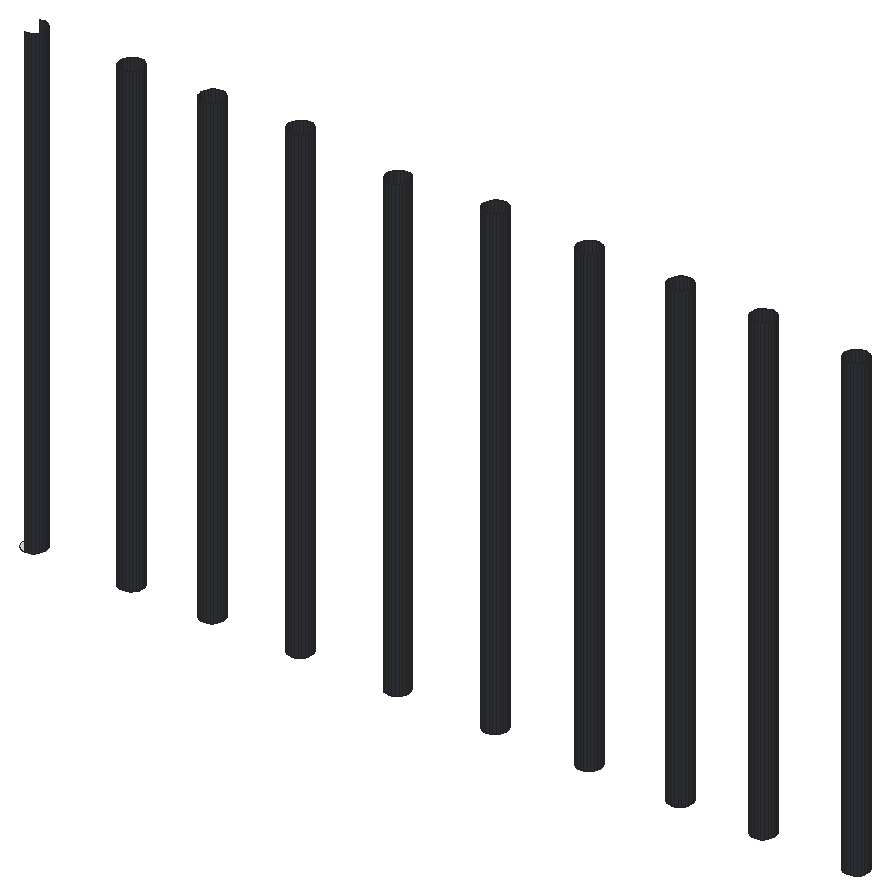
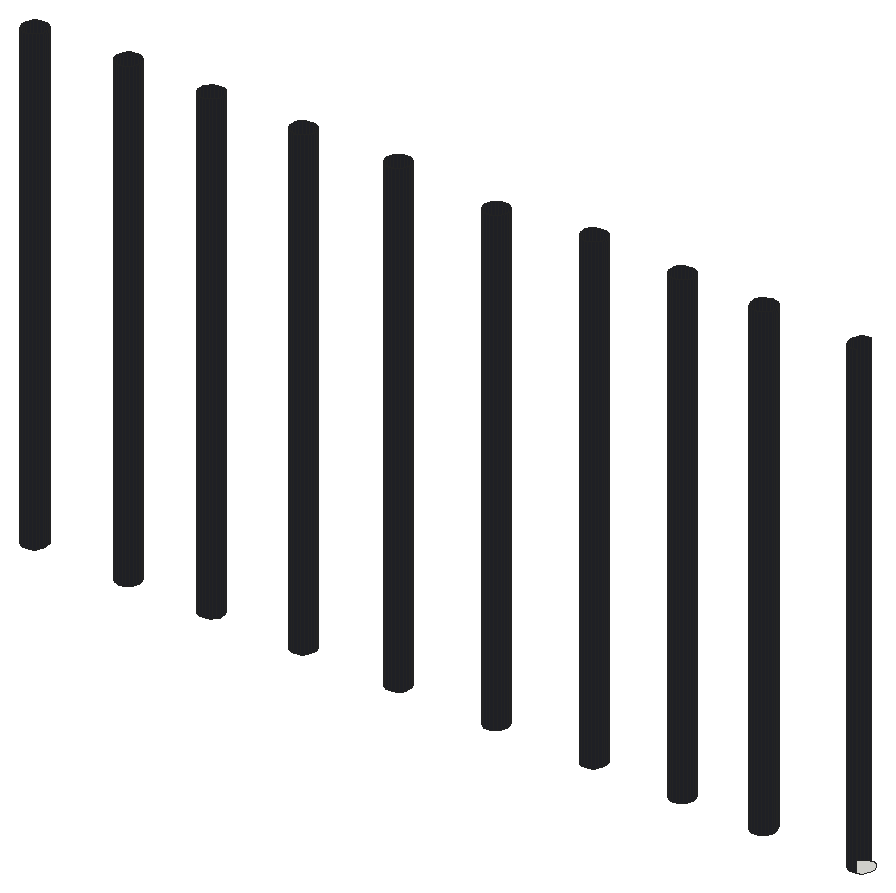
# SketchUp Ruby script. Lengths in inches.
U = 1.inch
M = Sketchup.active_model
def pt(a) = Geom::Point3d.new(a.map { |v| v * U })
def face(e, loops, mat)
  f = e.add_face(loops[0].map { |a| pt(a) })
  loops[1..].each { |l| e.add_face(l.map { |a| pt(a) }).erase! }
  f.material = f.back_material = mat if mat
  f
end
# faces: each face lists its corners as indices into pts; further lists are holes
def faces(e, pts, list, mat = nil) = list.each { |f| face(e, (f[0].is_a?(Array) ? f : [f]).map { |l| l.map { |i| pts[i] } }, mat) }
# xy, xz, yz: faces in a plane at the given z, y or x. An outline is a flat list of corners, or four numbers for a rectangle; further outlines are holes
def ring(l) = l.size == 4 ? [[l[0], l[1]], [l[2], l[1]], [l[2], l[3]], [l[0], l[3]]] : l.each_slice(2).to_a
def flat(e, list, mat, &to3) = list.each { |f| face(e, (f[0].is_a?(Array) ? f : [f]).map { |l| ring(l).map { |u, v| to3.(u, v) } }, mat) }
def xy(e, z, list, mat = nil) = flat(e, list, mat) { |x, y| [x, y, z] }
def xz(e, y, list, mat = nil) = flat(e, list, mat) { |x, z| [x, y, z] }
def yz(e, x, list, mat = nil) = flat(e, list, mat) { |y, z| [x, y, z] }
def lines(e, pts, list) = list.each { |a, b| e.add_line(pt(pts[a]), pt(pts[b])) }
# prism: a flat outline (further loops are holes) pulled along v
def prism(e, loops, v, mat = nil)
  f = face(e, loops, mat); d = Geom::Vector3d.new(v.map { |x| x * U })
  f.pushpull(f.normal.samedirection?(d) ? d.length : -d.length)
end
def box(e, o, s, mat = nil) = prism(e, [[o, [o[0] + s[0], o[1], o[2]], [o[0] + s[0], o[1] + s[1], o[2]], [o[0], o[1] + s[1], o[2]]]], [0, 0, s[2]], mat)
def at(x, y, z, deg = 0) = Geom::Transformation.translation(pt([x, y, z])) * Geom::Transformation.rotation(ORIGIN, Z_AXIS, deg.degrees)
def axes(o, x, y, z) = Geom::Transformation.new([*x, 0, *y, 0, *z, 0, *pt(o).to_a, 1])
def part(name) = M.definitions.add(name)
# library, detail: a bought-in or finely detailed component or shape, given as its bounding box
def library(name, o, s) = part(name).tap { |d| box(d.entities, o, s) }
def detail(e, o, s) = box(e.add_group.entities, o, s)
def put(e, d, t, mat = nil) = e.add_instance(d, t).tap { |i| i.material = mat if mat }
def group(e, t, mat = nil) = e.add_group.tap { |g| g.transformation = t; g.material = mat if mat }.entities
root = M.entities
M.materials.add("[Formica Laminate Dark]").color = [50, 53, 60]
xy(root,1179.9375,[[1326.55,797.03,1324.75,797.27,1323.08,797.96,1321.64,799.06,1320.54,800.5,1319.84,802.17,1319.61,803.97,1319.84,805.77,1320.54,807.4375,1321.64,808.875,1323.08,809.98,1324.75,810.67,1326.55,810.91,1328.34,810.67,1330.01,809.98,1331.45,808.875,1332.55,807.4375,1333.25,805.77,1333.48,803.97,1333.25,802.17,1332.55,800.5,1331.45,799.06,1330.01,797.96,1328.34,797.27],[1386.05,797.03,1384.25,797.27,1382.58,797.96,1381.14,799.06,1380.04,800.5,1379.34,802.17,1379.11,803.97,1379.34,805.77,1380.04,807.4375,1381.14,808.875,1382.58,809.98,1384.25,810.67,1386.05,810.91,1387.84,810.67,1389.51,809.98,1390.95,808.875,1392.05,807.4375,1392.75,805.77,1392.98,803.97,1392.75,802.17,1392.05,800.5,1390.95,799.06,1389.51,797.96,1387.84,797.27],[1435.55,797.03,1433.75,797.27,1432.08,797.96,1430.64,799.06,1429.54,800.5,1428.84,802.17,1428.61,803.97,1428.84,805.77,1429.54,807.4375,1430.64,808.875,1432.08,809.98,1433.75,810.67,1435.55,810.91,1437.34,810.67,1439.01,809.98,1440.45,808.875,1441.55,807.4375,1442.25,805.77,1442.48,803.97,1442.25,802.17,1441.55,800.5,1440.45,799.06,1439.01,797.96,1437.34,797.27],[1489.3,797.03,1487.5,797.27,1485.83,797.96,1484.39,799.06,1483.29,800.5,1482.59,802.17,1482.36,803.97,1482.59,805.77,1483.29,807.4375,1484.39,808.875,1485.83,809.98,1487.5,810.67,1489.3,810.91,1491.09,810.67,1492.76,809.98,1494.2,808.875,1495.3,807.4375,1496,805.77,1496.23,803.97,1496,802.17,1495.3,800.5,1494.2,799.06,1492.76,797.96,1491.09,797.27],[1548.73,797.03,1546.9375,797.27,1545.26,797.96,1543.83,799.06,1542.73,800.5,1542.03,802.17,1541.8,803.97,1542.03,805.77,1542.73,807.4375,1543.83,808.875,1545.26,809.98,1546.9375,810.67,1548.73,810.91,1550.53,810.67,1552.2,809.98,1553.64,808.875,1554.74,807.4375,1555.43,805.77,1555.67,803.97,1555.43,802.17,1554.74,800.5,1553.64,799.06,1552.2,797.96,1550.53,797.27],
  [1608.3,797.03,1606.5,797.27,1604.83,797.96,1603.39,799.06,1602.29,800.5,1601.59,802.17,1601.36,803.97,1601.59,805.77,1602.29,807.4375,1603.39,808.875,1604.83,809.98,1606.5,810.67,1608.3,810.91,1610.09,810.67,1611.76,809.98,1613.2,808.875,1614.3,807.4375,1615,805.77,1615.23,803.97,1615,802.17,1614.3,800.5,1613.2,799.06,1611.76,797.96,1610.09,797.27],[1665.86,797.03,1664.0625,797.27,1662.39,797.96,1660.95,799.06,1659.85,800.5,1659.16,802.17,1658.92,803.97,1659.16,805.77,1659.85,807.4375,1660.95,808.875,1662.39,809.98,1664.0625,810.67,1665.86,810.91,1667.65,810.67,1669.33,809.98,1670.76,808.875,1671.87,807.4375,1672.56,805.77,1672.8,803.97,1672.56,802.17,1671.87,800.5,1670.76,799.06,1669.33,797.96,1667.65,797.27],[1721.48,797.03,1719.6875,797.27,1718.01,797.96,1716.58,799.06,1715.48,800.5,1714.78,802.17,1714.55,803.97,1714.78,805.77,1715.48,807.4375,1716.58,808.875,1718.01,809.98,1719.6875,810.67,1721.48,810.91,1723.28,810.67,1724.95,809.98,1726.39,808.875,1727.49,807.4375,1728.18,805.77,1728.42,803.97,1728.18,802.17,1727.49,800.5,1726.39,799.06,1724.95,797.96,1723.28,797.27],[1772.17,797.03,1770.375,797.27,1768.7,797.96,1767.27,799.06,1766.16,800.5,1765.47,802.17,1765.23,803.97,1765.47,805.77,1766.16,807.4375,1767.27,808.875,1768.7,809.98,1770.375,810.67,1772.17,810.91,1773.97,810.67,1775.64,809.98,1777.08,808.875,1778.18,807.4375,1778.87,805.77,1779.11,803.97,1778.87,802.17,1778.18,800.5,1777.08,799.06,1775.64,797.96,1773.97,797.27],[1828.92,797.03,1827.125,797.27,1825.45,797.96,1824.02,799.06,1822.91,800.5,1822.22,802.17,1821.98,803.97,1822.22,805.77,1822.91,807.4375,1824.02,808.875,1825.45,809.98,1827.125,810.67,1828.92,810.91,1830.72,810.67,1832.39,809.98,1833.83,808.875,1834.93,807.4375,1835.62,805.77,1835.86,803.97,1835.62,802.17,1834.93,800.5,1833.83,799.06,1832.39,797.96,1830.72,797.27]])
p = [[1326.55,797.03,1179.9375],[1328.34,797.27,1179.9375],[1328.34,797.27,1464.6875],[1326.55,797.03,1464.6875],[1384.25,797.27,1179.9375],[1386.05,797.03,1179.9375],
  [1386.05,797.03,1464.6875],[1384.25,797.27,1464.6875],[1387.84,797.27,1179.9375],[1387.84,797.27,1464.6875],[1433.75,797.27,1179.9375],[1435.55,797.03,1179.9375],
  [1435.55,797.03,1464.6875],[1433.75,797.27,1464.6875],[1437.34,797.27,1179.9375],[1437.34,797.27,1464.6875],[1487.5,797.27,1179.9375],[1489.3,797.03,1179.9375],
  [1489.3,797.03,1466.5],[1487.5,797.27,1466.5],[1491.09,797.27,1179.9375],[1491.09,797.27,1466.5],[1546.9375,797.27,1179.9375],[1548.73,797.03,1179.9375],
  [1548.73,797.03,1460],[1546.9375,797.27,1460],[1550.53,797.27,1179.9375],[1550.53,797.27,1460],[1606.5,797.27,1179.9375],[1608.3,797.03,1179.9375],
  [1608.3,797.03,1464.6875],[1606.5,797.27,1464.6875],[1610.09,797.27,1179.9375],[1610.09,797.27,1464.6875],[1664.0625,797.27,1179.9375],[1665.86,797.03,1179.9375],
  [1665.86,797.03,1462.7],[1664.0625,797.27,1462.7],[1667.65,797.27,1179.9375],[1667.65,797.27,1462.7],[1719.6875,797.27,1179.9375],[1721.48,797.03,1179.9375],
  [1721.48,797.03,1462.7],[1719.6875,797.27,1462.7],[1723.28,797.27,1179.9375],[1723.28,797.27,1462.7],[1770.375,797.27,1179.9375],[1772.17,797.03,1179.9375],
  [1772.17,797.03,1462.7],[1770.375,797.27,1462.7],[1773.97,797.27,1179.9375],[1773.97,797.27,1462.7],[1827.125,797.27,1179.9375],[1828.92,797.03,1179.9375],
  [1828.92,797.03,1460.3125],[1827.125,797.27,1460.3125],[1830.72,797.27,1179.9375],[1830.72,797.27,1460.3125],[1330.01,797.96,1179.9375],[1330.01,797.96,1464.6875],
  [1382.58,797.96,1179.9375],[1382.58,797.96,1464.6875],[1389.51,797.96,1179.9375],[1389.51,797.96,1464.6875],[1432.08,797.96,1179.9375],[1432.08,797.96,1464.6875],
  [1439.01,797.96,1179.9375],[1439.01,797.96,1464.6875],[1485.83,797.96,1179.9375],[1485.83,797.96,1466.5],[1492.76,797.96,1179.9375],[1492.76,797.96,1466.5],
  [1545.26,797.96,1179.9375],[1545.26,797.96,1460],[1552.2,797.96,1179.9375],[1552.2,797.96,1460],[1604.83,797.96,1179.9375],[1604.83,797.96,1464.6875],
  [1611.76,797.96,1179.9375],[1611.76,797.96,1464.6875],[1662.39,797.96,1179.9375],[1662.39,797.96,1462.7],[1669.33,797.96,1179.9375],[1669.33,797.96,1462.7],
  [1718.01,797.96,1179.9375],[1718.01,797.96,1462.7],[1724.95,797.96,1179.9375],[1724.95,797.96,1462.7],[1768.7,797.96,1179.9375],[1768.7,797.96,1462.7],
  [1775.64,797.96,1179.9375],[1775.64,797.96,1462.7],[1825.45,797.96,1179.9375],[1825.45,797.96,1460.3125],[1832.39,797.96,1179.9375],[1832.39,797.96,1460.3125],
  [1331.45,799.06,1179.9375],[1331.45,799.06,1464.6875],[1381.14,799.06,1179.9375],[1381.14,799.06,1464.6875],[1390.95,799.06,1179.9375],[1390.95,799.06,1464.6875],
  [1430.64,799.06,1179.9375],[1430.64,799.06,1464.6875],[1440.45,799.06,1179.9375],[1440.45,799.06,1464.6875],[1484.39,799.06,1179.9375],[1484.39,799.06,1466.5],
  [1494.2,799.06,1179.9375],[1494.2,799.06,1466.5],[1543.83,799.06,1179.9375],[1543.83,799.06,1460],[1553.64,799.06,1179.9375],[1553.64,799.06,1460],
  [1603.39,799.06,1179.9375],[1603.39,799.06,1464.6875],[1613.2,799.06,1179.9375],[1613.2,799.06,1464.6875],[1660.95,799.06,1179.9375],[1660.95,799.06,1462.7],
  [1670.76,799.06,1179.9375],[1670.76,799.06,1462.7],[1716.58,799.06,1179.9375],[1716.58,799.06,1462.7],[1726.39,799.06,1179.9375],[1726.39,799.06,1462.7],
  [1767.27,799.06,1179.9375],[1767.27,799.06,1462.7],[1777.08,799.06,1179.9375],[1777.08,799.06,1462.7],[1824.02,799.06,1179.9375],[1824.02,799.06,1460.3125],
  [1833.83,799.06,1179.9375],[1833.83,799.06,1460.3125],[1332.55,800.5,1179.9375],[1332.55,800.5,1464.6875],[1380.04,800.5,1179.9375],[1380.04,800.5,1464.6875],
  [1392.05,800.5,1179.9375],[1392.05,800.5,1464.6875],[1429.54,800.5,1179.9375],[1429.54,800.5,1464.6875],[1441.55,800.5,1179.9375],[1441.55,800.5,1464.6875],
  [1483.29,800.5,1179.9375],[1483.29,800.5,1466.5],[1495.3,800.5,1179.9375],[1495.3,800.5,1466.5],[1542.73,800.5,1179.9375],[1542.73,800.5,1460],
  [1554.74,800.5,1179.9375],[1554.74,800.5,1460],[1602.29,800.5,1179.9375],[1602.29,800.5,1464.6875],[1614.3,800.5,1179.9375],[1614.3,800.5,1464.6875],
  [1659.85,800.5,1179.9375],[1659.85,800.5,1462.7],[1671.87,800.5,1179.9375],[1671.87,800.5,1462.7],[1715.48,800.5,1179.9375],[1715.48,800.5,1462.7],
  [1727.49,800.5,1179.9375],[1727.49,800.5,1462.7],[1766.16,800.5,1179.9375],[1766.16,800.5,1462.7],[1778.18,800.5,1179.9375],[1778.18,800.5,1462.7],
  [1822.91,800.5,1179.9375],[1822.91,800.5,1460.3125],[1834.93,800.5,1179.9375],[1834.93,800.5,1460.3125],[1333.25,802.17,1179.9375],[1333.25,802.17,1464.6875],
  [1379.34,802.17,1179.9375],[1379.34,802.17,1464.6875],[1392.75,802.17,1179.9375],[1392.75,802.17,1464.6875],[1428.84,802.17,1179.9375],[1428.84,802.17,1464.6875],
  [1442.25,802.17,1179.9375],[1442.25,802.17,1464.6875],[1482.59,802.17,1179.9375],[1482.59,802.17,1466.5],[1496,802.17,1179.9375],[1496,802.17,1466.5],
  [1542.03,802.17,1179.9375],[1542.03,802.17,1460],[1555.43,802.17,1179.9375],[1555.43,802.17,1460],[1601.59,802.17,1179.9375],[1601.59,802.17,1464.6875],
  [1615,802.17,1179.9375],[1615,802.17,1464.6875],[1659.16,802.17,1179.9375],[1659.16,802.17,1462.7],[1672.56,802.17,1179.9375],[1672.56,802.17,1462.7],
  [1714.78,802.17,1179.9375],[1714.78,802.17,1462.7],[1728.18,802.17,1179.9375],[1728.18,802.17,1462.7],[1765.47,802.17,1179.9375],[1765.47,802.17,1462.7],
  [1778.87,802.17,1179.9375],[1778.87,802.17,1462.7],[1822.22,802.17,1179.9375],[1822.22,802.17,1460.3125],[1835.62,802.17,1179.9375],[1835.62,802.17,1460.3125],
  [1333.48,803.97,1179.9375],[1333.48,803.97,1464.6875],[1379.11,803.97,1179.9375],[1379.11,803.97,1464.6875],[1392.98,803.97,1179.9375],[1392.98,803.97,1464.6875],
  [1428.61,803.97,1179.9375],[1428.61,803.97,1464.6875],[1442.48,803.97,1179.9375],[1442.48,803.97,1464.6875],[1482.36,803.97,1179.9375],[1482.36,803.97,1466.5],
  [1496.23,803.97,1179.9375],[1496.23,803.97,1466.5],[1541.8,803.97,1179.9375],[1541.8,803.97,1460],[1555.67,803.97,1179.9375],[1555.67,803.97,1460],
  [1601.36,803.97,1179.9375],[1601.36,803.97,1464.6875],[1615.23,803.97,1179.9375],[1615.23,803.97,1464.6875],[1658.92,803.97,1179.9375],[1658.92,803.97,1462.7],
  [1672.8,803.97,1179.9375],[1672.8,803.97,1462.7],[1714.55,803.97,1179.9375],[1714.55,803.97,1462.7],[1728.42,803.97,1179.9375],[1728.42,803.97,1462.7],
  [1765.23,803.97,1179.9375],[1765.23,803.97,1462.7],[1779.11,803.97,1179.9375],[1779.11,803.97,1462.7],[1821.98,803.97,1179.9375],[1821.98,803.97,1460.3125],
  [1835.86,803.97,1179.9375],[1835.86,803.97,1460.3125],[1333.25,805.77,1179.9375],[1333.25,805.77,1464.6875],[1379.34,805.77,1179.9375],[1379.34,805.77,1464.6875],
  [1392.75,805.77,1179.9375],[1392.75,805.77,1464.6875],[1428.84,805.77,1179.9375],[1428.84,805.77,1464.6875],[1442.25,805.77,1179.9375],[1442.25,805.77,1464.6875],
  [1482.59,805.77,1179.9375],[1482.59,805.77,1466.5],[1496,805.77,1179.9375],[1496,805.77,1466.5],[1542.03,805.77,1179.9375],[1542.03,805.77,1460],
  [1555.43,805.77,1179.9375],[1555.43,805.77,1460],[1601.59,805.77,1179.9375],[1601.59,805.77,1464.6875],[1615,805.77,1179.9375],[1615,805.77,1464.6875],
  [1659.16,805.77,1179.9375],[1659.16,805.77,1462.7],[1672.56,805.77,1179.9375],[1672.56,805.77,1462.7],[1714.78,805.77,1179.9375],[1714.78,805.77,1462.7],
  [1728.18,805.77,1179.9375],[1728.18,805.77,1462.7],[1765.47,805.77,1179.9375],[1765.47,805.77,1462.7],[1778.87,805.77,1179.9375],[1778.87,805.77,1462.7],
  [1822.22,805.77,1179.9375],[1822.22,805.77,1460.3125],[1835.62,805.77,1179.9375],[1835.62,805.77,1460.3125],[1332.55,807.4375,1179.9375],[1332.55,807.4375,1464.6875],
  [1380.04,807.4375,1179.9375],[1380.04,807.4375,1464.6875],[1392.05,807.4375,1179.9375],[1392.05,807.4375,1464.6875],[1429.54,807.4375,1179.9375],[1429.54,807.4375,1464.6875],
  [1441.55,807.4375,1179.9375],[1441.55,807.4375,1464.6875],[1483.29,807.4375,1179.9375],[1483.29,807.4375,1466.5],[1495.3,807.4375,1179.9375],[1495.3,807.4375,1466.5],
  [1542.73,807.4375,1179.9375],[1542.73,807.4375,1460],[1554.74,807.4375,1179.9375],[1554.74,807.4375,1460],[1602.29,807.4375,1179.9375],[1602.29,807.4375,1464.6875],
  [1614.3,807.4375,1179.9375],[1614.3,807.4375,1464.6875],[1659.85,807.4375,1179.9375],[1659.85,807.4375,1462.7],[1671.87,807.4375,1179.9375],[1671.87,807.4375,1462.7],
  [1715.48,807.4375,1179.9375],[1715.48,807.4375,1462.7],[1727.49,807.4375,1179.9375],[1727.49,807.4375,1462.7],[1766.16,807.4375,1179.9375],[1766.16,807.4375,1462.7],
  [1778.18,807.4375,1179.9375],[1778.18,807.4375,1462.7],[1822.91,807.4375,1179.9375],[1822.91,807.4375,1460.3125],[1834.93,807.4375,1179.9375],[1834.93,807.4375,1460.3125],
  [1331.45,808.875,1179.9375],[1331.45,808.875,1464.6875],[1381.14,808.875,1179.9375],[1381.14,808.875,1464.6875],[1390.95,808.875,1179.9375],[1390.95,808.875,1464.6875],
  [1430.64,808.875,1179.9375],[1430.64,808.875,1464.6875],[1440.45,808.875,1179.9375],[1440.45,808.875,1464.6875],[1484.39,808.875,1179.9375],[1484.39,808.875,1466.5],
  [1494.2,808.875,1179.9375],[1494.2,808.875,1466.5],[1543.83,808.875,1179.9375],[1543.83,808.875,1460],[1553.64,808.875,1179.9375],[1553.64,808.875,1460],
  [1603.39,808.875,1179.9375],[1603.39,808.875,1464.6875],[1613.2,808.875,1179.9375],[1613.2,808.875,1464.6875],[1660.95,808.875,1179.9375],[1660.95,808.875,1462.7],
  [1670.76,808.875,1179.9375],[1670.76,808.875,1462.7],[1716.58,808.875,1179.9375],[1716.58,808.875,1462.7],[1726.39,808.875,1179.9375],[1726.39,808.875,1462.7],
  [1767.27,808.875,1179.9375],[1767.27,808.875,1462.7],[1777.08,808.875,1179.9375],[1777.08,808.875,1462.7],[1824.02,808.875,1179.9375],[1824.02,808.875,1460.3125],
  [1833.83,808.875,1179.9375],[1833.83,808.875,1460.3125],[1330.01,809.98,1179.9375],[1330.01,809.98,1464.6875],[1382.58,809.98,1179.9375],[1382.58,809.98,1464.6875],
  [1389.51,809.98,1179.9375],[1389.51,809.98,1464.6875],[1432.08,809.98,1179.9375],[1432.08,809.98,1464.6875],[1439.01,809.98,1179.9375],[1439.01,809.98,1464.6875],
  [1485.83,809.98,1179.9375],[1485.83,809.98,1466.5],[1492.76,809.98,1179.9375],[1492.76,809.98,1466.5],[1545.26,809.98,1179.9375],[1545.26,809.98,1460],
  [1552.2,809.98,1179.9375],[1552.2,809.98,1460],[1604.83,809.98,1179.9375],[1604.83,809.98,1464.6875],[1611.76,809.98,1179.9375],[1611.76,809.98,1464.6875],
  [1662.39,809.98,1179.9375],[1662.39,809.98,1462.7],[1669.33,809.98,1179.9375],[1669.33,809.98,1462.7],[1718.01,809.98,1179.9375],[1718.01,809.98,1462.7],
  [1724.95,809.98,1179.9375],[1724.95,809.98,1462.7],[1768.7,809.98,1179.9375],[1768.7,809.98,1462.7],[1775.64,809.98,1179.9375],[1775.64,809.98,1462.7],
  [1825.45,809.98,1179.9375],[1825.45,809.98,1460.3125],[1832.39,809.98,1179.9375],[1832.39,809.98,1460.3125],[1328.34,810.67,1179.9375],[1328.34,810.67,1464.6875],
  [1384.25,810.67,1179.9375],[1384.25,810.67,1464.6875],[1387.84,810.67,1179.9375],[1387.84,810.67,1464.6875],[1433.75,810.67,1179.9375],[1433.75,810.67,1464.6875],
  [1437.34,810.67,1179.9375],[1437.34,810.67,1464.6875],[1487.5,810.67,1179.9375],[1487.5,810.67,1466.5],[1491.09,810.67,1179.9375],[1491.09,810.67,1466.5],
  [1546.9375,810.67,1179.9375],[1546.9375,810.67,1460],[1550.53,810.67,1179.9375],[1550.53,810.67,1460],[1606.5,810.67,1179.9375],[1606.5,810.67,1464.6875],
  [1610.09,810.67,1179.9375],[1610.09,810.67,1464.6875],[1664.0625,810.67,1179.9375],[1664.0625,810.67,1462.7],[1667.65,810.67,1179.9375],[1667.65,810.67,1462.7],
  [1719.6875,810.67,1179.9375],[1719.6875,810.67,1462.7],[1723.28,810.67,1179.9375],[1723.28,810.67,1462.7],[1770.375,810.67,1179.9375],[1770.375,810.67,1462.7],
  [1773.97,810.67,1179.9375],[1773.97,810.67,1462.7],[1827.125,810.67,1179.9375],[1827.125,810.67,1460.3125],[1830.72,810.67,1179.9375],[1830.72,810.67,1460.3125],
  [1326.55,810.91,1179.9375],[1324.75,810.67,1179.9375],[1324.75,810.67,1464.6875],[1325.87,810.82,1464.6875],[1326.55,810.91,1464.6875],[1327.23,810.82,1464.6875],
  [1386.05,810.91,1179.9375],[1385.37,810.82,1464.6875],[1386.05,810.91,1464.6875],[1386.73,810.82,1464.6875],[1435.55,810.91,1179.9375],[1434.87,810.82,1464.6875],
  [1435.55,810.91,1464.6875],[1436.23,810.82,1464.6875],[1489.3,810.91,1179.9375],[1489.3,810.91,1466.5],[1548.73,810.91,1179.9375],[1548.73,810.91,1460],
  [1608.3,810.91,1179.9375],[1607.62,810.82,1464.6875],[1608.3,810.91,1464.6875],[1608.98,810.82,1464.6875],[1665.86,810.91,1179.9375],[1665.86,810.91,1462.7],
  [1721.48,810.91,1179.9375],[1721.48,810.91,1462.7],[1772.17,810.91,1179.9375],[1772.17,810.91,1462.7],[1828.92,810.91,1179.9375],[1828.92,810.91,1460.3125]]
faces(root,p,[[0,1,2,3],[4,5,6,7],[5,8,9,6],[10,11,12,13],[11,14,15,12],[16,17,18,19],[17,20,21,18],[22,23,24,25],
  [23,26,27,24],[28,29,30,31],[29,32,33,30],[34,35,36,37],[35,38,39,36],[40,41,42,43],[41,44,45,42],[46,47,48,49],
  [47,50,51,48],[52,53,54,55],[53,56,57,54],[1,58,59,2],[60,4,7,61],[8,62,63,9],[64,10,13,65],[14,66,67,15],
  [68,16,19,69],[20,70,71,21],[72,22,25,73],[26,74,75,27],[76,28,31,77],[32,78,79,33],[80,34,37,81],[38,82,83,39],
  [84,40,43,85],[44,86,87,45],[88,46,49,89],[50,90,91,51],[92,52,55,93],[56,94,95,57],[58,96,97,59],[98,60,61,99],
  [62,100,101,63],[102,64,65,103],[66,104,105,67],[106,68,69,107],[70,108,109,71],[110,72,73,111],[74,112,113,75],[114,76,77,115],
  [78,116,117,79],[118,80,81,119],[82,120,121,83],[122,84,85,123],[86,124,125,87],[126,88,89,127],[90,128,129,91],[130,92,93,131],
  [94,132,133,95],[96,134,135,97],[136,98,99,137],[100,138,139,101],[140,102,103,141],[104,142,143,105],[144,106,107,145],[108,146,147,109],
  [148,110,111,149],[112,150,151,113],[152,114,115,153],[116,154,155,117],[156,118,119,157],[120,158,159,121],[160,122,123,161],[124,162,163,125],
  [164,126,127,165],[128,166,167,129],[168,130,131,169],[132,170,171,133],[134,172,173,135],[174,136,137,175],[138,176,177,139],[178,140,141,179],
  [142,180,181,143],[182,144,145,183],[146,184,185,147],[186,148,149,187],[150,188,189,151],[190,152,153,191],[154,192,193,155],[194,156,157,195],
  [158,196,197,159],[198,160,161,199],[162,200,201,163],[202,164,165,203],[166,204,205,167],[206,168,169,207],[170,208,209,171],[172,210,211,173],
  [212,174,175,213],[176,214,215,177],[216,178,179,217],[180,218,219,181],[220,182,183,221],[184,222,223,185],[224,186,187,225],[188,226,227,189],
  [228,190,191,229],[192,230,231,193],[232,194,195,233],[196,234,235,197],[236,198,199,237],[200,238,239,201],[240,202,203,241],[204,242,243,205],
  [244,206,207,245],[208,246,247,209],[210,248,249,211],[250,212,213,251],[214,252,253,215],[254,216,217,255],[218,256,257,219],[258,220,221,259],
  [222,260,261,223],[262,224,225,263],[226,264,265,227],[266,228,229,267],[230,268,269,231],[270,232,233,271],[234,272,273,235],[274,236,237,275],
  [238,276,277,239],[278,240,241,279],[242,280,281,243],[282,244,245,283],[246,284,285,247],[248,286,287,249],[288,250,251,289],[252,290,291,253],
  [292,254,255,293],[256,294,295,257],[296,258,259,297],[260,298,299,261],[300,262,263,301],[264,302,303,265],[304,266,267,305],[268,306,307,269],
  [308,270,271,309],[272,310,311,273],[312,274,275,313],[276,314,315,277],[316,278,279,317],[280,318,319,281],[320,282,283,321],[284,322,323,285],
  [286,324,325,287],[326,288,289,327],[290,328,329,291],[330,292,293,331],[294,332,333,295],[334,296,297,335],[298,336,337,299],[338,300,301,339],
  [302,340,341,303],[342,304,305,343],[306,344,345,307],[346,308,309,347],[310,348,349,311],[350,312,313,351],[314,352,353,315],[354,316,317,355],
  [318,356,357,319],[358,320,321,359],[322,360,361,323],[324,362,363,325],[364,326,327,365],[328,366,367,329],[368,330,331,369],[332,370,371,333],
  [372,334,335,373],[336,374,375,337],[376,338,339,377],[340,378,379,341],[380,342,343,381],[344,382,383,345],[384,346,347,385],[348,386,387,349],
  [388,350,351,389],[352,390,391,353],[392,354,355,393],[356,394,395,357],[396,358,359,397],[360,398,399,361],[362,400,401,363],[402,364,365,403],
  [366,404,405,367],[406,368,369,407],[370,408,409,371],[410,372,373,411],[374,412,413,375],[414,376,377,415],[378,416,417,379],[418,380,381,419],
  [382,420,421,383],[422,384,385,423],[386,424,425,387],[426,388,389,427],[390,428,429,391],[430,392,393,431],[394,432,433,395],[434,396,397,435],
  [398,436,437,399],[438,439,440,441,442],[400,438,442,443,401],[444,402,403,445,446],[404,444,446,447,405],[448,406,407,449,450],[408,448,450,451,409],[452,410,411,453],
  [412,452,453,413],[454,414,415,455],[416,454,455,417],[456,418,419,457,458],[420,456,458,459,421],[460,422,423,461],[424,460,461,425],[462,426,427,463],
  [428,462,463,429],[464,430,431,465],[432,464,465,433],[466,434,435,467],[436,466,467,437]],"[Formica Laminate Dark]")
